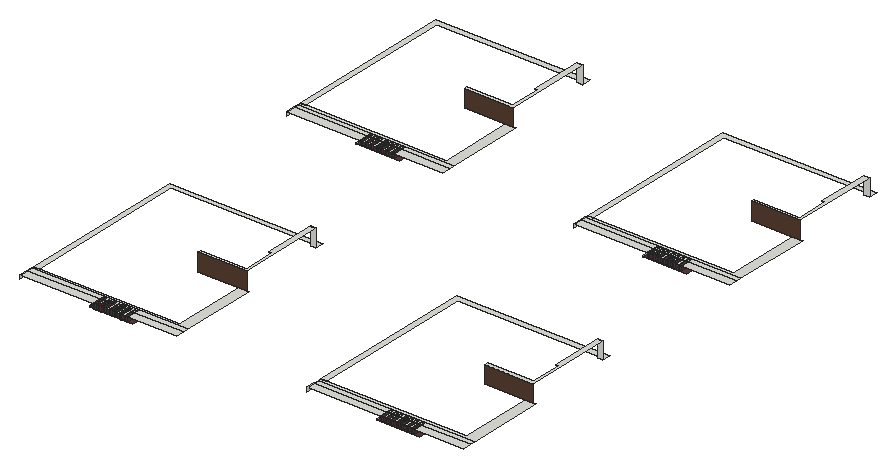
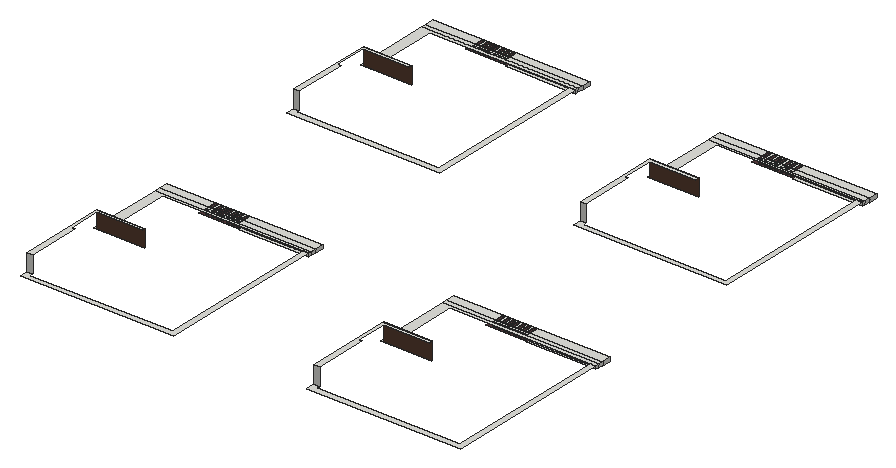
# SketchUp Ruby script. Lengths in inches.
U = 1.inch
M = Sketchup.active_model
def pt(a) = Geom::Point3d.new(a.map { |v| v * U })
def face(e, loops, mat)
  f = e.add_face(loops[0].map { |a| pt(a) })
  loops[1..].each { |l| e.add_face(l.map { |a| pt(a) }).erase! }
  f.material = f.back_material = mat if mat
  f
end
# faces: each face lists its corners as indices into pts; further lists are holes
def faces(e, pts, list, mat = nil) = list.each { |f| face(e, (f[0].is_a?(Array) ? f : [f]).map { |l| l.map { |i| pts[i] } }, mat) }
# xy, xz, yz: faces in a plane at the given z, y or x. An outline is a flat list of corners, or four numbers for a rectangle; further outlines are holes
def ring(l) = l.size == 4 ? [[l[0], l[1]], [l[2], l[1]], [l[2], l[3]], [l[0], l[3]]] : l.each_slice(2).to_a
def flat(e, list, mat, &to3) = list.each { |f| face(e, (f[0].is_a?(Array) ? f : [f]).map { |l| ring(l).map { |u, v| to3.(u, v) } }, mat) }
def xy(e, z, list, mat = nil) = flat(e, list, mat) { |x, y| [x, y, z] }
def xz(e, y, list, mat = nil) = flat(e, list, mat) { |x, z| [x, y, z] }
def yz(e, x, list, mat = nil) = flat(e, list, mat) { |y, z| [x, y, z] }
def lines(e, pts, list) = list.each { |a, b| e.add_line(pt(pts[a]), pt(pts[b])) }
# prism: a flat outline (further loops are holes) pulled along v
def prism(e, loops, v, mat = nil)
  f = face(e, loops, mat); d = Geom::Vector3d.new(v.map { |x| x * U })
  f.pushpull(f.normal.samedirection?(d) ? d.length : -d.length)
end
def box(e, o, s, mat = nil) = prism(e, [[o, [o[0] + s[0], o[1], o[2]], [o[0] + s[0], o[1] + s[1], o[2]], [o[0], o[1] + s[1], o[2]]]], [0, 0, s[2]], mat)
def at(x, y, z, deg = 0) = Geom::Transformation.translation(pt([x, y, z])) * Geom::Transformation.rotation(ORIGIN, Z_AXIS, deg.degrees)
def axes(o, x, y, z) = Geom::Transformation.new([*x, 0, *y, 0, *z, 0, *pt(o).to_a, 1])
def part(name) = M.definitions.add(name)
# library, detail: a bought-in or finely detailed component or shape, given as its bounding box
def library(name, o, s) = part(name).tap { |d| box(d.entities, o, s) }
def detail(e, o, s) = box(e.add_group.entities, o, s)
def put(e, d, t, mat = nil) = e.add_instance(d, t).tap { |i| i.material = mat if mat }
def group(e, t, mat = nil) = e.add_group.tap { |g| g.transformation = t; g.material = mat if mat }.entities
root = M.entities
M.materials.add("[Granite Brown]").color = [89, 59, 61]
M.materials.add("[Granite Brown]1").color = [89, 63, 50]
xy(root,1801.625,[[557.4,1763.25,557.88,1799.9375],[[557.88,1763.25,741.54,1822.9375],[573.13,1766.43,584.19,1816.55],[595.19,1766.43,606.25,1816.55],[616.25,1766.43,627.31,1816.55],[639.94,1766.43,651,1816.55],[659.38,1766.43,670.44,1816.55],[681.63,1766.43,692.69,1816.55],[706,1766.43,717.06,1816.55]],[1775.59,1763.25,1776.07,1799.9375],[[1776.07,1763.25,1959.73,1822.9375],[1791.31,1766.43,1802.38,1816.55],[1813.38,1766.43,1824.44,1816.55],[1834.44,1766.43,1845.5,1816.55],[1858.13,1766.43,1869.19,1816.55],[1877.56,1766.43,1888.63,1816.55],[1899.81,1766.43,1910.88,1816.55],[1924.19,1766.43,1935.25,1816.55]],[557.4,1799.9375,557.88,1822.9375],
  [1775.59,1799.9375,1776.07,1822.9375],[557.4,3177.9375,557.88,3214.625],[[557.88,3177.9375,741.54,3237.625],[573.13,3181.12,584.19,3231.24],[595.19,3181.12,606.25,3231.24],[616.25,3181.12,627.31,3231.24],[639.94,3181.12,651,3231.24],[659.38,3181.12,670.44,3231.24],[681.63,3181.12,692.69,3231.24],[706,3181.12,717.06,3231.24]],[1775.59,3177.9375,1776.07,3214.625],[[1776.07,3177.9375,1959.73,3237.625],[1791.31,3181.12,1802.38,3231.24],[1813.38,3181.12,1824.44,3231.24],[1834.44,3181.12,1845.5,3231.24],[1858.13,3181.12,1869.19,3231.24],[1877.56,3181.12,1888.63,3231.24],[1899.81,3181.12,1910.88,3231.24],[1924.19,3181.12,1935.25,3231.24]],
  [557.4,3214.625,557.88,3237.625],[1775.59,3214.625,1776.07,3237.625]],"[Granite Brown]")
xy(root,1805.3125,[[557.22,1763.25,557.4,1778.3125],[1775.4,1763.25,1775.59,1778.3125],[523.04,1799.9375,557.4,1822.9375],[1741.23,1799.9375,1775.59,1822.9375],[557.22,3177.9375,557.4,3193],
  [1775.4,3177.9375,1775.59,3193],[523.04,3214.625,557.4,3237.625],[1741.23,3214.625,1775.59,3237.625]])
xy(root,1807.33,[[262.875,1799.9375,319.53,1822.9375],[319.53,1799.9375,557.4,1822.9375],[1481.0625,1799.9375,1537.72,1822.9375],[1537.72,1799.9375,1775.59,1822.9375],[262.875,1822.9375,285.875,1835.8125],
  [285.875,1822.9375,557.4,1835.8125],[1481.0625,1822.9375,1504.0625,1835.8125],[1504.0625,1822.9375,1775.59,1835.8125],[262.875,3214.625,319.53,3237.625],[319.53,3214.625,557.4,3237.625],
  [1481.0625,3214.625,1537.72,3237.625],[1537.72,3214.625,1775.59,3237.625],[262.875,3237.625,285.875,3250.5],[285.875,3237.625,557.4,3250.5],[1481.0625,3237.625,1504.0625,3250.5],
  [1504.0625,3237.625,1775.59,3250.5]])
xy(root,1808.75,[[407.44,1806.5625,431.33,1822.9375],[1625.63,1806.5625,1649.52,1822.9375],[407.44,3221.25,431.33,3237.625],[1625.63,3221.25,1649.52,3237.625]])
xy(root,1821.625,[[262.875,1763.25,925.6875,1763.25,925.6875,1799.9375,717.06,1799.9375,717.06,1766.43,706,1766.43,706,1799.9375,692.69,1799.9375,692.69,1766.43,681.63,1766.43,681.63,1799.9375,670.44,1799.9375,670.44,1766.43,659.38,1766.43,659.38,1799.9375,651,1799.9375,651,1766.43,639.94,1766.43,639.94,1799.9375,627.31,1799.9375,627.31,1766.43,616.25,1766.43,616.25,1799.9375,606.25,1799.9375,606.25,1766.43,595.19,1766.43,595.19,1799.9375,584.19,1799.9375,584.19,1766.43,573.13,1766.43,573.13,1799.9375,262.875,1799.9375],[1481.0625,1763.25,2143.875,1763.25,2143.875,1799.9375,1935.25,1799.9375,1935.25,1766.43,1924.19,1766.43,1924.19,1799.9375,1910.88,1799.9375,1910.88,1766.43,1899.81,1766.43,1899.81,1799.9375,1888.63,1799.9375,1888.63,1766.43,1877.56,1766.43,1877.56,1799.9375,1869.19,1799.9375,1869.19,1766.43,1858.13,1766.43,1858.13,1799.9375,1845.5,1799.9375,1845.5,1766.43,1834.44,1766.43,1834.44,1799.9375,1824.44,1799.9375,1824.44,1766.43,1813.38,1766.43,1813.38,1799.9375,1802.38,1799.9375,1802.38,1766.43,1791.31,1766.43,1791.31,1799.9375,1481.0625,1799.9375],[262.875,1799.9375,573.13,1799.9375,573.13,1816.55,584.19,1816.55,584.19,1799.9375,595.19,1799.9375,595.19,1816.55,606.25,1816.55,606.25,1799.9375,616.25,1799.9375,616.25,1816.55,627.31,1816.55,627.31,1799.9375,639.94,1799.9375,639.94,1816.55,651,1816.55,651,1799.9375,659.38,1799.9375,659.38,1816.55,670.44,1816.55,670.44,1799.9375,681.63,1799.9375,681.63,1816.55,692.69,1816.55,692.69,1799.9375,706,1799.9375,706,1816.55,717.06,1816.55,717.06,1799.9375,925.6875,1799.9375,925.6875,1822.9375,262.875,1822.9375],[573.13,1799.9375,584.19,1816.55],[595.19,1799.9375,606.25,1816.55],
  [616.25,1799.9375,627.31,1816.55],[639.94,1799.9375,651,1816.55],[659.38,1799.9375,670.44,1816.55],[681.63,1799.9375,692.69,1816.55],[706,1799.9375,717.06,1816.55],
  [1481.0625,1799.9375,1791.31,1799.9375,1791.31,1816.55,1802.38,1816.55,1802.38,1799.9375,1813.38,1799.9375,1813.38,1816.55,1824.44,1816.55,1824.44,1799.9375,1834.44,1799.9375,1834.44,1816.55,1845.5,1816.55,1845.5,1799.9375,1858.13,1799.9375,1858.13,1816.55,1869.19,1816.55,1869.19,1799.9375,1877.56,1799.9375,1877.56,1816.55,1888.63,1816.55,1888.63,1799.9375,1899.81,1799.9375,1899.81,1816.55,1910.88,1816.55,1910.88,1799.9375,1924.19,1799.9375,1924.19,1816.55,1935.25,1816.55,1935.25,1799.9375,2143.875,1799.9375,2143.875,1822.9375,1481.0625,1822.9375],[1791.31,1799.9375,1802.38,1816.55],[1813.38,1799.9375,1824.44,1816.55],[1834.44,1799.9375,1845.5,1816.55],[1858.13,1799.9375,1869.19,1816.55],
  [1877.56,1799.9375,1888.63,1816.55],[1899.81,1799.9375,1910.88,1816.55],[1924.19,1799.9375,1935.25,1816.55],[262.875,1822.9375,925.6875,1822.9375,925.6875,2148.83,883.05,2148.83,883.05,1835.8125,262.875,1835.8125],[1481.0625,1822.9375,2143.875,1822.9375,2143.875,2148.83,2101.24,2148.83,2101.24,1835.8125,1481.0625,1835.8125],
  [262.875,1835.8125,285.875,1835.8125,285.875,2531.375,890.875,2531.375,890.875,2518.89,913.875,2518.89,913.875,2554.375,262.875,2554.375],[1481.0625,1835.8125,1504.0625,1835.8125,1504.0625,2531.375,2109.0625,2531.375,2109.0625,2518.89,2132.0625,2518.89,2132.0625,2554.375,1481.0625,2554.375],[262.875,3177.9375,925.6875,3177.9375,925.6875,3214.625,717.06,3214.625,717.06,3181.12,706,3181.12,706,3214.625,692.69,3214.625,692.69,3181.12,681.63,3181.12,681.63,3214.625,670.44,3214.625,670.44,3181.12,659.38,3181.12,659.38,3214.625,651,3214.625,651,3181.12,639.94,3181.12,639.94,3214.625,627.31,3214.625,627.31,3181.12,616.25,3181.12,616.25,3214.625,606.25,3214.625,606.25,3181.12,595.19,3181.12,595.19,3214.625,584.19,3214.625,584.19,3181.12,573.13,3181.12,573.13,3214.625,262.875,3214.625],[1481.0625,3177.9375,2143.875,3177.9375,2143.875,3214.625,1935.25,3214.625,1935.25,3181.12,1924.19,3181.12,1924.19,3214.625,1910.88,3214.625,1910.88,3181.12,1899.81,3181.12,1899.81,3214.625,1888.63,3214.625,1888.63,3181.12,1877.56,3181.12,1877.56,3214.625,1869.19,3214.625,1869.19,3181.12,1858.13,3181.12,1858.13,3214.625,1845.5,3214.625,1845.5,3181.12,1834.44,3181.12,1834.44,3214.625,1824.44,3214.625,1824.44,3181.12,1813.38,3181.12,1813.38,3214.625,1802.38,3214.625,1802.38,3181.12,1791.31,3181.12,1791.31,3214.625,1481.0625,3214.625],[262.875,3214.625,573.13,3214.625,573.13,3231.24,584.19,3231.24,584.19,3214.625,595.19,3214.625,595.19,3231.24,606.25,3231.24,606.25,3214.625,616.25,3214.625,616.25,3231.24,627.31,3231.24,627.31,3214.625,639.94,3214.625,639.94,3231.24,651,3231.24,651,3214.625,659.38,3214.625,659.38,3231.24,670.44,3231.24,670.44,3214.625,681.63,3214.625,681.63,3231.24,692.69,3231.24,692.69,3214.625,706,3214.625,706,3231.24,717.06,3231.24,717.06,3214.625,925.6875,3214.625,925.6875,3237.625,262.875,3237.625],
  [573.13,3214.625,584.19,3231.24],[595.19,3214.625,606.25,3231.24],[616.25,3214.625,627.31,3231.24],[639.94,3214.625,651,3231.24],[659.38,3214.625,670.44,3231.24],
  [681.63,3214.625,692.69,3231.24],[706,3214.625,717.06,3231.24],[1481.0625,3214.625,1791.31,3214.625,1791.31,3231.24,1802.38,3231.24,1802.38,3214.625,1813.38,3214.625,1813.38,3231.24,1824.44,3231.24,1824.44,3214.625,1834.44,3214.625,1834.44,3231.24,1845.5,3231.24,1845.5,3214.625,1858.13,3214.625,1858.13,3231.24,1869.19,3231.24,1869.19,3214.625,1877.56,3214.625,1877.56,3231.24,1888.63,3231.24,1888.63,3214.625,1899.81,3214.625,1899.81,3231.24,1910.88,3231.24,1910.88,3214.625,1924.19,3214.625,1924.19,3231.24,1935.25,3231.24,1935.25,3214.625,2143.875,3214.625,2143.875,3237.625,1481.0625,3237.625],[1791.31,3214.625,1802.38,3231.24],[1813.38,3214.625,1824.44,3231.24],
  [1834.44,3214.625,1845.5,3231.24],[1858.13,3214.625,1869.19,3231.24],[1877.56,3214.625,1888.63,3231.24],[1899.81,3214.625,1910.88,3231.24],[1924.19,3214.625,1935.25,3231.24],
  [262.875,3237.625,925.6875,3237.625,925.6875,3563.51,883.05,3563.51,883.05,3250.5,262.875,3250.5],[1481.0625,3237.625,2143.875,3237.625,2143.875,3563.51,2101.24,3563.51,2101.24,3250.5,1481.0625,3250.5],[262.875,3250.5,285.875,3250.5,285.875,3946.0625,890.875,3946.0625,890.875,3933.57,913.875,3933.57,913.875,3969.0625,262.875,3969.0625],[1481.0625,3250.5,1504.0625,3250.5,1504.0625,3946.0625,2109.0625,3946.0625,2109.0625,3933.57,2132.0625,3933.57,2132.0625,3969.0625,1481.0625,3969.0625]])
xy(root,1821.625,[[573.13,1766.43,584.19,1799.9375],[595.19,1766.43,606.25,1799.9375],[616.25,1766.43,627.31,1799.9375],[639.94,1766.43,651,1799.9375],[659.38,1766.43,670.44,1799.9375],
  [681.63,1766.43,692.69,1799.9375],[706,1766.43,717.06,1799.9375],[1791.31,1766.43,1802.38,1799.9375],[1813.38,1766.43,1824.44,1799.9375],[1834.44,1766.43,1845.5,1799.9375],
  [1858.13,1766.43,1869.19,1799.9375],[1877.56,1766.43,1888.63,1799.9375],[1899.81,1766.43,1910.88,1799.9375],[1924.19,1766.43,1935.25,1799.9375],[573.13,3181.12,584.19,3214.625],
  [595.19,3181.12,606.25,3214.625],[616.25,3181.12,627.31,3214.625],[639.94,3181.12,651,3214.625],[659.38,3181.12,670.44,3214.625],[681.63,3181.12,692.69,3214.625],
  [706,3181.12,717.06,3214.625],[1791.31,3181.12,1802.38,3214.625],[1813.38,3181.12,1824.44,3214.625],[1834.44,3181.12,1845.5,3214.625],[1858.13,3181.12,1869.19,3214.625],
  [1877.56,3181.12,1888.63,3214.625],[1899.81,3181.12,1910.88,3214.625],[1924.19,3181.12,1935.25,3214.625]],"[Granite Brown]")
xy(root,1895.25,[[708.18,2148.83,913.875,2148.83,913.875,2518.89,890.875,2518.89,890.875,2295.875,903.5,2295.875,903.5,2162.73,708.18,2162.73],[1926.36,2148.83,2132.0625,2148.83,2132.0625,2518.89,2109.0625,2518.89,2109.0625,2295.875,2121.6875,2295.875,2121.6875,2162.73,1926.36,2162.73],[708.18,3563.51,913.875,3563.51,913.875,3933.57,890.875,3933.57,890.875,3710.5625,903.5,3710.5625,903.5,3577.41,708.18,3577.41],[1926.36,3563.51,2132.0625,3563.51,2132.0625,3933.57,2109.0625,3933.57,2109.0625,3710.5625,2121.6875,3710.5625,2121.6875,3577.41,1926.36,3577.41]])
xz(root,1766.43,[[573.13,1801.625,584.19,1821.625],[595.19,1801.625,606.25,1821.625],[616.25,1801.625,627.31,1821.625],[639.94,1801.625,651,1821.625],[659.38,1801.625,670.44,1821.625],
  [681.63,1801.625,692.69,1821.625],[706,1801.625,717.06,1821.625],[1791.31,1801.625,1802.38,1821.625],[1813.38,1801.625,1824.44,1821.625],[1834.44,1801.625,1845.5,1821.625],
  [1858.13,1801.625,1869.19,1821.625],[1877.56,1801.625,1888.63,1821.625],[1899.81,1801.625,1910.88,1821.625],[1924.19,1801.625,1935.25,1821.625]],"[Granite Brown]")
xz(root,1799.9375,[[319.53,1805.3125,557.4,1807.33],[1537.72,1805.3125,1775.59,1807.33]])
xz(root,1816.55,[[573.13,1801.625,584.19,1821.625],[595.19,1801.625,606.25,1821.625],[616.25,1801.625,627.31,1821.625],[639.94,1801.625,651,1821.625],[659.38,1801.625,670.44,1821.625],
  [681.63,1801.625,692.69,1821.625],[706,1801.625,717.06,1821.625],[1791.31,1801.625,1802.38,1821.625],[1813.38,1801.625,1824.44,1821.625],[1834.44,1801.625,1845.5,1821.625],
  [1858.13,1801.625,1869.19,1821.625],[1877.56,1801.625,1888.63,1821.625],[1899.81,1801.625,1910.88,1821.625],[1924.19,1801.625,1935.25,1821.625]],"[Granite Brown]")
xz(root,1835.8125,[[262.875,1807.33,285.875,1821.625],[1481.0625,1807.33,1504.0625,1821.625]])
xz(root,2148.83,[[708.18,1821.625,913.875,1895.25],[1926.36,1821.625,2132.0625,1895.25]],"[Granite Brown]1")
xz(root,2518.89,[[890.875,1821.625,913.875,1895.25],[2109.0625,1821.625,2132.0625,1895.25]])
xz(root,3181.12,[[573.13,1801.625,584.19,1821.625],[595.19,1801.625,606.25,1821.625],[616.25,1801.625,627.31,1821.625],[639.94,1801.625,651,1821.625],[659.38,1801.625,670.44,1821.625],
  [681.63,1801.625,692.69,1821.625],[706,1801.625,717.06,1821.625],[1791.31,1801.625,1802.38,1821.625],[1813.38,1801.625,1824.44,1821.625],[1834.44,1801.625,1845.5,1821.625],
  [1858.13,1801.625,1869.19,1821.625],[1877.56,1801.625,1888.63,1821.625],[1899.81,1801.625,1910.88,1821.625],[1924.19,1801.625,1935.25,1821.625]],"[Granite Brown]")
xz(root,3214.625,[[319.53,1805.3125,557.4,1807.33],[1537.72,1805.3125,1775.59,1807.33]])
xz(root,3231.24,[[573.13,1801.625,584.19,1821.625],[595.19,1801.625,606.25,1821.625],[616.25,1801.625,627.31,1821.625],[639.94,1801.625,651,1821.625],[659.38,1801.625,670.44,1821.625],
  [681.63,1801.625,692.69,1821.625],[706,1801.625,717.06,1821.625],[1791.31,1801.625,1802.38,1821.625],[1813.38,1801.625,1824.44,1821.625],[1834.44,1801.625,1845.5,1821.625],
  [1858.13,1801.625,1869.19,1821.625],[1877.56,1801.625,1888.63,1821.625],[1899.81,1801.625,1910.88,1821.625],[1924.19,1801.625,1935.25,1821.625]],"[Granite Brown]")
xz(root,3250.5,[[262.875,1807.33,285.875,1821.625],[1481.0625,1807.33,1504.0625,1821.625]])
xz(root,3563.51,[[708.18,1821.625,913.875,1895.25],[1926.36,1821.625,2132.0625,1895.25]],"[Granite Brown]1")
xz(root,3933.57,[[890.875,1821.625,913.875,1895.25],[2109.0625,1821.625,2132.0625,1895.25]])
yz(root,262.875,[[1763.25,1805.3125,1799.9375,1821.625],[3177.9375,1805.3125,3214.625,1821.625],[1799.9375,1807.33,1822.9375,1821.625],[1822.9375,1807.33,1835.8125,1821.625],[3214.625,1807.33,3237.625,1821.625],
  [3237.625,1807.33,3250.5,1821.625]])
yz(root,557.4,[[1763.25,1801.625,1799.9375,1805.3125],[1799.9375,1801.625,1822.9375,1805.3125],[3177.9375,1801.625,3214.625,1805.3125],[3214.625,1801.625,3237.625,1805.3125],[1799.9375,1805.3125,1822.9375,1807.33],
  [3214.625,1805.3125,3237.625,1807.33]])
yz(root,573.13,[[1766.43,1801.625,1816.55,1821.625],[3181.12,1801.625,3231.24,1821.625]],"[Granite Brown]")
yz(root,584.19,[[1766.43,1801.625,1816.55,1821.625],[3181.12,1801.625,3231.24,1821.625]],"[Granite Brown]")
yz(root,595.19,[[1766.43,1801.625,1816.55,1821.625],[3181.12,1801.625,3231.24,1821.625]],"[Granite Brown]")
yz(root,606.25,[[1766.43,1801.625,1816.55,1821.625],[3181.12,1801.625,3231.24,1821.625]],"[Granite Brown]")
yz(root,616.25,[[1766.43,1801.625,1816.55,1821.625],[3181.12,1801.625,3231.24,1821.625]],"[Granite Brown]")
yz(root,627.31,[[1766.43,1801.625,1816.55,1821.625],[3181.12,1801.625,3231.24,1821.625]],"[Granite Brown]")
yz(root,639.94,[[1766.43,1801.625,1816.55,1821.625],[3181.12,1801.625,3231.24,1821.625]],"[Granite Brown]")
yz(root,651,[[1766.43,1801.625,1816.55,1821.625],[3181.12,1801.625,3231.24,1821.625]],"[Granite Brown]")
yz(root,659.38,[[1766.43,1801.625,1816.55,1821.625],[3181.12,1801.625,3231.24,1821.625]],"[Granite Brown]")
yz(root,670.44,[[1766.43,1801.625,1816.55,1821.625],[3181.12,1801.625,3231.24,1821.625]],"[Granite Brown]")
yz(root,681.63,[[1766.43,1801.625,1816.55,1821.625],[3181.12,1801.625,3231.24,1821.625]],"[Granite Brown]")
yz(root,692.69,[[1766.43,1801.625,1816.55,1821.625],[3181.12,1801.625,3231.24,1821.625]],"[Granite Brown]")
yz(root,706,[[1766.43,1801.625,1816.55,1821.625],[3181.12,1801.625,3231.24,1821.625]],"[Granite Brown]")
yz(root,717.06,[[1766.43,1801.625,1816.55,1821.625],[3181.12,1801.625,3231.24,1821.625]],"[Granite Brown]")
yz(root,1481.0625,[[1763.25,1805.3125,1799.9375,1821.625],[3177.9375,1805.3125,3214.625,1821.625],[1799.9375,1807.33,1822.9375,1821.625],[1822.9375,1807.33,1835.8125,1821.625],[3214.625,1807.33,3237.625,1821.625],
  [3237.625,1807.33,3250.5,1821.625]])
yz(root,1775.59,[[1763.25,1801.625,1799.9375,1805.3125],[1799.9375,1801.625,1822.9375,1805.3125],[3177.9375,1801.625,3214.625,1805.3125],[3214.625,1801.625,3237.625,1805.3125],[1799.9375,1805.3125,1822.9375,1807.33],
  [3214.625,1805.3125,3237.625,1807.33]])
yz(root,1791.31,[[1766.43,1801.625,1816.55,1821.625],[3181.12,1801.625,3231.24,1821.625]],"[Granite Brown]")
yz(root,1802.38,[[1766.43,1801.625,1816.55,1821.625],[3181.12,1801.625,3231.24,1821.625]],"[Granite Brown]")
yz(root,1813.38,[[1766.43,1801.625,1816.55,1821.625],[3181.12,1801.625,3231.24,1821.625]],"[Granite Brown]")
yz(root,1824.44,[[1766.43,1801.625,1816.55,1821.625],[3181.12,1801.625,3231.24,1821.625]],"[Granite Brown]")
yz(root,1834.44,[[1766.43,1801.625,1816.55,1821.625],[3181.12,1801.625,3231.24,1821.625]],"[Granite Brown]")
yz(root,1845.5,[[1766.43,1801.625,1816.55,1821.625],[3181.12,1801.625,3231.24,1821.625]],"[Granite Brown]")
yz(root,1858.13,[[1766.43,1801.625,1816.55,1821.625],[3181.12,1801.625,3231.24,1821.625]],"[Granite Brown]")
yz(root,1869.19,[[1766.43,1801.625,1816.55,1821.625],[3181.12,1801.625,3231.24,1821.625]],"[Granite Brown]")
yz(root,1877.56,[[1766.43,1801.625,1816.55,1821.625],[3181.12,1801.625,3231.24,1821.625]],"[Granite Brown]")
yz(root,1888.63,[[1766.43,1801.625,1816.55,1821.625],[3181.12,1801.625,3231.24,1821.625]],"[Granite Brown]")
yz(root,1899.81,[[1766.43,1801.625,1816.55,1821.625],[3181.12,1801.625,3231.24,1821.625]],"[Granite Brown]")
yz(root,1910.88,[[1766.43,1801.625,1816.55,1821.625],[3181.12,1801.625,3231.24,1821.625]],"[Granite Brown]")
yz(root,1924.19,[[1766.43,1801.625,1816.55,1821.625],[3181.12,1801.625,3231.24,1821.625]],"[Granite Brown]")
yz(root,1935.25,[[1766.43,1801.625,1816.55,1821.625],[3181.12,1801.625,3231.24,1821.625]],"[Granite Brown]")
p = [[407.65,1806.5625,1805.3125],[407.65,1822.9375,1805.3125],[407.44,1822.9375,1805.3125],[396.84,1822.9375,1805.37],[396.84,1806.5625,1805.37],[407.44,1806.5625,1805.3125],
  [1625.84,1806.5625,1805.3125],[1625.84,1822.9375,1805.3125],[1625.63,1822.9375,1805.3125],[1615.02,1822.9375,1805.37],[1615.02,1806.5625,1805.37],[1625.63,1806.5625,1805.3125],
  [407.65,3221.25,1805.3125],[407.65,3237.625,1805.3125],[407.44,3237.625,1805.3125],[396.84,3237.625,1805.37],[396.84,3221.25,1805.37],[407.44,3221.25,1805.3125],
  [1625.84,3221.25,1805.3125],[1625.84,3237.625,1805.3125],[1625.63,3237.625,1805.3125],[1615.02,3237.625,1805.37],[1615.02,3221.25,1805.37],[1625.63,3221.25,1805.3125],
  [1537.72,1799.9375,1805.3125],[1537.72,1781.8125,1805.3125],[1625.63,1822.9375,1807.33],[1625.63,1822.9375,1808.75],[319.53,1799.9375,1805.3125],[319.53,1781.8125,1805.3125],
  [407.44,1822.9375,1807.33],[407.44,1822.9375,1808.75],[1537.72,3214.625,1805.3125],[1537.72,3196.5,1805.3125],[1625.63,3237.625,1807.33],[1625.63,3237.625,1808.75],
  [407.44,3237.625,1807.33],[407.44,3237.625,1808.75],[319.53,3214.625,1805.3125],[319.53,3196.5,1805.3125]]
faces(root,p,[[0,1,2,3,4,5],[6,7,8,9,10,11],[12,13,14,15,16,17],[18,19,20,21,22,23]])
lines(root,p,[[24,25],[26,27],[28,29],[30,31],[32,33],[34,35],[36,37],[38,39]])
